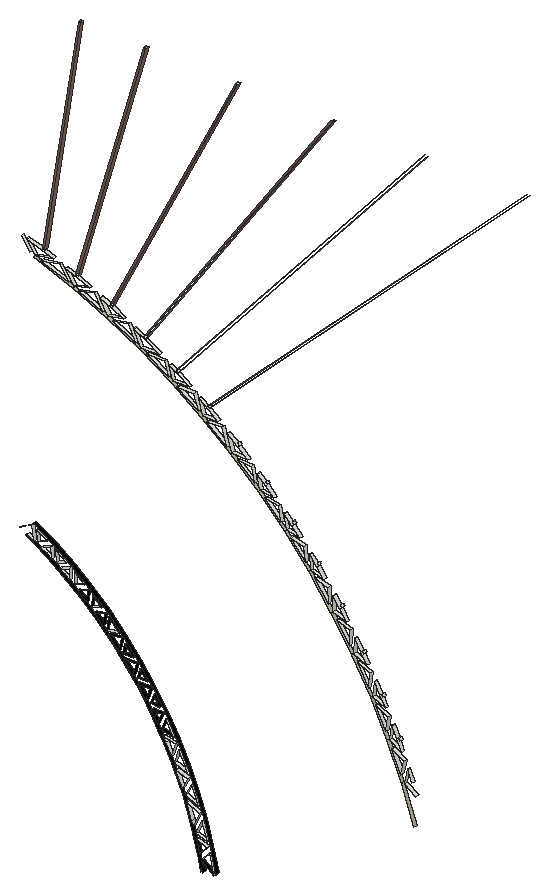
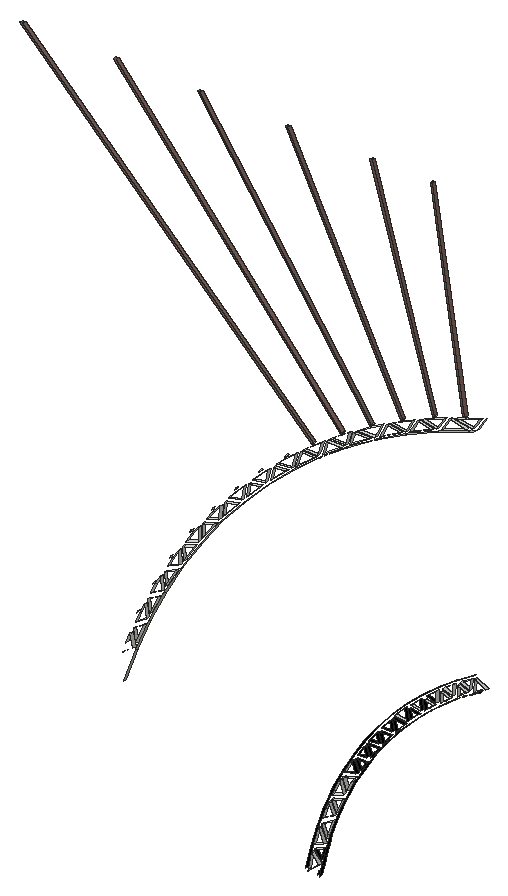
# SketchUp Ruby script. Lengths in inches.
U = 1.inch
M = Sketchup.active_model
def pt(a) = Geom::Point3d.new(a.map { |v| v * U })
def face(e, loops, mat)
  f = e.add_face(loops[0].map { |a| pt(a) })
  loops[1..].each { |l| e.add_face(l.map { |a| pt(a) }).erase! }
  f.material = f.back_material = mat if mat
  f
end
# faces: each face lists its corners as indices into pts; further lists are holes
def faces(e, pts, list, mat = nil) = list.each { |f| face(e, (f[0].is_a?(Array) ? f : [f]).map { |l| l.map { |i| pts[i] } }, mat) }
# xy, xz, yz: faces in a plane at the given z, y or x. An outline is a flat list of corners, or four numbers for a rectangle; further outlines are holes
def ring(l) = l.size == 4 ? [[l[0], l[1]], [l[2], l[1]], [l[2], l[3]], [l[0], l[3]]] : l.each_slice(2).to_a
def flat(e, list, mat, &to3) = list.each { |f| face(e, (f[0].is_a?(Array) ? f : [f]).map { |l| ring(l).map { |u, v| to3.(u, v) } }, mat) }
def xy(e, z, list, mat = nil) = flat(e, list, mat) { |x, y| [x, y, z] }
def xz(e, y, list, mat = nil) = flat(e, list, mat) { |x, z| [x, y, z] }
def yz(e, x, list, mat = nil) = flat(e, list, mat) { |y, z| [x, y, z] }
def lines(e, pts, list) = list.each { |a, b| e.add_line(pt(pts[a]), pt(pts[b])) }
# prism: a flat outline (further loops are holes) pulled along v
def prism(e, loops, v, mat = nil)
  f = face(e, loops, mat); d = Geom::Vector3d.new(v.map { |x| x * U })
  f.pushpull(f.normal.samedirection?(d) ? d.length : -d.length)
end
def box(e, o, s, mat = nil) = prism(e, [[o, [o[0] + s[0], o[1], o[2]], [o[0] + s[0], o[1] + s[1], o[2]], [o[0], o[1] + s[1], o[2]]]], [0, 0, s[2]], mat)
def at(x, y, z, deg = 0) = Geom::Transformation.translation(pt([x, y, z])) * Geom::Transformation.rotation(ORIGIN, Z_AXIS, deg.degrees)
def axes(o, x, y, z) = Geom::Transformation.new([*x, 0, *y, 0, *z, 0, *pt(o).to_a, 1])
def part(name) = M.definitions.add(name)
# library, detail: a bought-in or finely detailed component or shape, given as its bounding box
def library(name, o, s) = part(name).tap { |d| box(d.entities, o, s) }
def detail(e, o, s) = box(e.add_group.entities, o, s)
def put(e, d, t, mat = nil) = e.add_instance(d, t).tap { |i| i.material = mat if mat }
def group(e, t, mat = nil) = e.add_group.tap { |g| g.transformation = t; g.material = mat if mat }.entities
root = M.entities
M.materials.add("Tafisa-Terrarossa-PM780-4K").color = [148, 117, 107]
M.materials.add("Uniboard-L19-Putty-4K").color = [187, 181, 160]
M.materials.add("[Color M09]").color = [0, 0, 0]
xy(root,59.17,[[115.33,138,116.01,138.16]],"[Color M09]")
xy(root,59.41,[[115.33,138,115.86,138.16]],"[Color M09]")
xy(root,60.06,[[114.61,138,115.28,138.16]],"[Color M09]")
xy(root,60.3,[[114.58,138,115.15,138.16]],"[Color M09]")
xy(root,72.82,[[119,138,119.8,138.16]])
xy(root,73.01,[[118.79,138,119.59,138.16]])
xy(root,73.9,[[117.43,138,118.31,138.16]])
xy(root,74.1,[[117.19,138,118.07,138.16]])
xy(root,74.89,[[115.81,138,116.77,138.16]])
xy(root,75.08,[[115.51,138,116.49,138.16]])
xy(root,89.29,[[112.22,138,112.34,138.16],[115.67,138,115.8,138.16],[120.5,138,120.63,138.16],[125.54,138,125.68,138.16]])
yz(root,110.47,[[138,77.92,138.16,77.94]])
yz(root,112.11,[[138,77.33,138.16,77.35]])
yz(root,118.75,[[138,53.89,138.16,53.9]])
p = [[118.68,138,51.44],[118.55,138,52.01],[118.55,138.16,52.01],[118.68,138.16,51.44],[118.72,138,52.02],[119.36,138,51.48],
  [119.36,138.16,51.48],[118.72,138.16,52.02],[118.75,138,51.68],[118.8,138,51.47],[118.8,138.16,51.47],[118.75,138.16,51.68],
  [119.34,138,51.57],[119.34,138.16,51.57],[119.14,138,52.5],[119.14,138.16,52.5],[119.2,138,52.77],[119.47,138,51.6],
  [119.47,138.16,51.6],[119.2,138.16,52.77],[118.42,138,52.57],[118.42,138.16,52.57],[118.54,138,52.6],[118.62,138,52.28],
  [118.62,138.16,52.28],[118.54,138.16,52.6],[119,138,52.72],[119,138.16,52.72],[118.26,138,53.125],[118.26,138.16,53.125],
  [118.45,138,52.92],[118.45,138.16,52.92],[118.87,138,53.93],[118.87,138.16,53.93],[118.43,138,53.2],[119.02,138,52.97],
  [119.02,138.16,52.97],[118.43,138.16,53.2],[118.75,138,53.89],[118.75,138.16,53.89],[118.1,138,53.68],[118.1,138.16,53.68],
  [118.75,138,53.9],[118.75,138.16,53.9],[118.22,138,53.72],[118.29,138,53.48],[118.29,138.16,53.48],[118.22,138.16,53.72],
  [118.6,138,54.17],[118.6,138.16,54.17],[117.71,138,54.77],[117.71,138.16,54.77],[117.93,138,54.51],[117.93,138.16,54.51],
  [118.76,138,54.22],[118.76,138.16,54.22],[118.46,138,55.0625],[118.46,138.16,55.0625],[117.875,138,54.82],[118.54,138,54.48],
  [118.54,138.16,54.48],[117.875,138.16,54.82],[118.34,138,55.02],[118.34,138.16,55.02],[117.25,138,55.83],[117.25,138.16,55.83],
  [118.18,138,55.4],[118.18,138.16,55.4],[117.38,138,55.83],[117.72,138,55.05],[117.72,138.16,55.05],[117.38,138.16,55.83],
  [118.01,138,55.62],[118.01,138.16,55.62],[118.1875,138,55.6875],[118.1875,138.16,55.6875],[117.98,138,56.17],[117.98,138.16,56.17],
  [117.14,138,56.04],[117.14,138.16,56.04],[117.3,138,56.12],[117.96,138,55.89],[117.96,138.16,55.89],[117.3,138.16,56.12],
  [117.87,138,56.12],[117.87,138.16,56.12],[116.73,138,56.86],[116.73,138.16,56.86],[117.53,138,56.79],[117.53,138.16,56.79],
  [117.5,138,57.1],[117.5,138.16,57.1],[116.84,138,56.92],[117.12,138,56.36],[117.12,138.16,56.36],[116.84,138.16,56.92],
  [117.34,138,57.02],[117.34,138.16,57.02],[116.43,138,57.35],[116.43,138.16,57.35],[116.6875,138,57.17],[116.6875,138.16,57.17],
  [117.43,138,57.24],[117.43,138.16,57.24],[116.82,138,58.28],[116.82,138.16,58.28],[116.6,138,57.44],[117.26,138,57.29],
  [117.26,138.16,57.29],[116.6,138.16,57.44],[116.84,138,58.01],[116.84,138.16,58.01],[116.14,138,57.85],[116.14,138.16,57.85],
  [129.91,138,57.52],[129.25,138,59.34],[129.25,138.16,59.34],[129.91,138.16,57.52],[116.24,138,57.92],[116.41,138,57.63],
  [116.41,138.16,57.63],[116.24,138.16,57.92],[116.64,138,58.17],[116.64,138.16,58.17],[115.82,138,58.33],[115.82,138.16,58.33],
  [116.06,138,58.19],[116.06,138.16,58.19],[115.49,138,58.81],[115.49,138.16,58.81],[116.14,138,59.28],[116.14,138.16,59.28],
  [116.02,138,58.47],[116.53,138,58.44],[116.53,138.16,58.44],[116.02,138.16,58.47],[116.1875,138,58.95],[116.1875,138.16,58.95],
  [115.57,138,58.86],[115.79,138,58.53],[115.79,138.16,58.53],[115.57,138.16,58.86],[116.01,138,59.17],[116.01,138.16,59.17],
  [115.14,138,59.26],[115.14,138.16,59.26],[115.33,138,59.17],[115.33,138.16,59.17],[129.39,138,59.39],[130,138,58.98],
  [130,138.16,58.98],[129.39,138.16,59.39],[114.78,138,59.72],[114.78,138.16,59.72],[115.4,138,60.23],[115.4,138.16,60.23],
  [128.48,138,61.11],[128.48,138.16,61.11],[115.48,138,59.89],[115.33,138,59.41],[115.33,138.16,59.41],[115.48,138.16,59.89],
  [115.86,138,59.41],[115.86,138.16,59.41],[129.55,138,60.11],[129.55,138.16,60.11],[114.85,138,59.78],[115.1,138,59.46],
  [115.1,138.16,59.46],[114.85,138.16,59.78],[115.28,138,60.06],[115.28,138.16,60.06],[129.79,138,59.55],[129.79,138.16,59.55],
  [114.4,138,60.15],[114.4,138.16,60.15],[128.75,138,60.8125],[129.21,138,59.73],[129.21,138.16,59.73],[128.75,138.16,60.8125],
  [129.375,138,60.44],[129.375,138.16,60.44],[114.61,138,60.06],[114.61,138.16,60.06],[114.02,138,60.58],[114.02,138.16,60.58],
  [114.61,138,61.13],[114.61,138.16,61.13],[114.6875,138,60.82],[114.58,138,60.3],[114.58,138.16,60.3],[114.6875,138.16,60.82],
  [115.15,138,60.3],[115.15,138.16,60.3],[114.09,138,60.65],[114.35,138,60.35],[114.35,138.16,60.35],[114.09,138.16,60.65],
  [114.49,138,61.02],[114.49,138.16,61.02],[113.61,138,60.99],[113.61,138.16,60.99],[113.81,138,60.93],[113.81,138.16,60.93],
  [128.62,138,61.18],[129.25,138,60.8],[129.25,138.16,60.8],[128.62,138.16,61.18],[129.01,138,61.36],[129.01,138.16,61.36],
  [113.2,138,61.4],[113.2,138.16,61.4],[113.82,138,61.79],[113.72,138,61.1],[113.72,138.16,61.1],[113.82,138.16,61.79],
  [114.41,138,61.2],[114.41,138.16,61.2],[113.75,138,61.99],[113.75,138.16,61.99],[127.6,138,62.84],[127.6,138.16,62.84],
  [128.74,138,61.9],[128.74,138.16,61.9],[113.29,138,61.5],[113.52,138,61.27],[113.52,138.16,61.27],[113.29,138.16,61.5],
  [113.6,138,61.82],[113.6,138.16,61.82],[129.125,138,61.41],[129.17,138,61.3],[129.17,138.16,61.3],[129.125,138.16,61.41],
  [112.77,138,61.78],[112.77,138.16,61.78],[113.05,138,61.71],[113.05,138.16,61.71],[127.89,138,62.55],[128.42,138,61.51],
  [128.42,138.16,61.51],[127.89,138.16,62.55],[128.54,138,62.23],[128.54,138.16,62.23],[112.34,138,62.16],[112.34,138.16,62.16],
  [112.96,138,62.51],[112.91,138,61.95],[112.91,138.16,61.95],[112.96,138.16,62.51],[113.47,138,62.0625],[113.47,138.16,62.0625],
  [112.85,138,62.78],[112.85,138.16,62.78],[112.42,138,62.27],[112.66,138,62.06],[112.66,138.16,62.06],[112.42,138.16,62.27],
  [112.7,138,62.61],[112.7,138.16,62.61],[111.88,138,62.52],[111.88,138.16,62.52],[112.17,138,62.46],[112.17,138.16,62.46],
  [111.42,138,62.87],[111.42,138.16,62.87],[127.74,138,62.91],[128.39,138,62.58],[128.39,138.16,62.58],[127.74,138.16,62.91],
  [128.12,138,63.12],[128.12,138.16,63.12],[112.02,138,63.26],[112.01,138,62.69],[112.01,138.16,62.69],[112.02,138.16,63.26],
  [112.5625,138,62.84],[112.5625,138.16,62.84],[111.5,138,62.98],[111.75,138,62.78],[111.75,138.16,62.78],[111.5,138.16,62.98],
  [111.76,138,63.34],[111.76,138.16,63.34],[111.9,138,63.52],[111.9,138.16,63.52],[126.62,138,64.5],[126.62,138.16,64.5],
  [110.95,138,63.2],[110.95,138.16,63.2],[127.81,138,63.64],[127.81,138.16,63.64],[111.24,138,63.16],[111.24,138.16,63.16],
  [128.23,138,63.18],[128.28,138,63.07],[128.28,138.16,63.07],[128.23,138.16,63.18],[110.47,138,63.52],[110.47,138.16,63.52],
  [126.92,138,64.24],[127.52,138,63.23],[127.52,138.16,63.23],[126.92,138.16,64.24],[127.59,138,63.95],[127.59,138.16,63.95],
  [111.04,138,63.94],[111.07,138,63.38],[111.07,138.16,63.38],[111.04,138.16,63.94],[111.61,138,63.5625],[111.61,138.16,63.5625],
  [109.97,138,63.82],[109.97,138.16,63.82],[110.54,138,63.63],[110.8,138,63.45],[110.8,138.16,63.45],[110.54,138.16,63.63],
  [110.78,138,64.01],[110.78,138.16,64.01],[110.9,138,64.2],[110.9,138.16,64.2],[110.26,138,63.8],[110.26,138.16,63.8],
  [109.47,138,64.11],[109.47,138.16,64.11],[109.52,138,64.18],[109.87,138,63.97],[109.87,138.16,63.97],[109.52,138.16,64.18],
  [109.79,138,64.6875],[109.79,138.16,64.6875],[110.02,138,64.57],[110.08,138,64],[110.08,138.16,64],[110.02,138.16,64.57],
  [110.61,138,64.22],[110.61,138.16,64.22],[109.86,138,64.8125],[109.86,138.16,64.8125],[126.75,138,64.58],[127.42,138,64.29],
  [127.42,138.16,64.29],[126.75,138.16,64.58],[127.11,138,64.8125],[127.11,138.16,64.8125],[109.15,138,64.37],[109.15,138.16,64.37],
  [125.53,138,66.1],[125.53,138.16,66.1],[126.77,138,65.32],[126.77,138.16,65.32],[127.22,138,64.88],[127.28,138,64.78],
  [127.28,138.16,64.78],[127.22,138.16,64.88],[125.85,138,65.86],[126.51,138,64.88],[126.51,138.16,64.88],[125.85,138.16,65.86],
  [126.53,138,65.61],[126.53,138.16,65.61],[125.65,138,66.19],[126.35,138,65.94],[126.35,138.16,65.94],[125.65,138.16,66.19],
  [126.01,138,66.44],[126.01,138.16,66.44],[124.35,138,67.63],[124.35,138.16,67.63],[125.63,138,66.92],[125.63,138.16,66.92],
  [124.68,138,67.41],[125.4,138,66.48],[125.4,138.16,66.48],[124.68,138.16,67.41],[125.38,138,67.21],[125.38,138.16,67.21],
  [126.03,138,66.61],[126.11,138,66.52],[126.11,138.16,66.52],[126.03,138.16,66.61],[126.06,138,66.625],[126.06,138.16,66.625],
  [124.46,138,67.73],[125.17,138,67.52],[125.17,138.16,67.52],[124.46,138.16,67.73],[124.8,138,68],[124.8,138.16,68],
  [123.07,138,69.08],[123.07,138.16,69.08],[124.4,138,68.46],[124.4,138.16,68.46],[123.41,138,68.88],[124.1875,138,68],
  [124.1875,138.16,68],[123.41,138.16,68.88],[124.12,138,68.72],[124.12,138.16,68.72],[124.8125,138,68.17],[124.89,138,68.08],
  [124.89,138.16,68.08],[124.8125,138.16,68.17],[124.84,138,68.1875],[124.84,138.16,68.1875],[123.18,138,69.18],[123.89,138,69.03],
  [123.89,138.16,69.03],[123.18,138.16,69.18],[123.49,138,69.48],[123.49,138.16,69.48],[121.7,138,70.45],[121.7,138.16,70.45],
  [123.06,138,69.91],[123.06,138.16,69.91],[122.06,138,70.27],[122.89,138,69.4375],[122.89,138.16,69.4375],[122.06,138.16,70.27],
  [122.78,138,70.16],[122.78,138.16,70.16],[123.5,138,69.65],[123.58,138,69.57],[123.58,138.16,69.57],[123.5,138.16,69.65],
  [123.52,138,69.67],[123.52,138.16,69.67],[120.25,138,71.73],[120.25,138.16,71.73],[121.8,138,70.56],[122.53,138,70.45],
  [122.53,138.16,70.45],[121.8,138.16,70.56],[122.1,138,70.875],[122.1,138.16,70.875],[121.64,138,71.28],[121.64,138.16,71.28],
  [120.61,138,71.57],[121.5,138,70.79],[121.5,138.16,70.79],[120.61,138.16,71.57],[121.34,138,71.5],[121.34,138.16,71.5],
  [122.12,138,71.0625],[122.09,138,71.05],[122.09,138.16,71.05],[122.12,138.16,71.0625],[122.18,138,70.97],[122.18,138.16,70.97],
  [118.72,138,72.91],[118.72,138.16,72.91],[120.32,138,71.82],[121.16,138,71.74],[121.16,138.16,71.74],[120.32,138.16,71.82],
  [120.64,138,72.2],[120.64,138.16,72.2],[120.06,138,72.65],[120.06,138.16,72.65],[119,138,72.82],[120.0625,138,71.99],
  [120.0625,138.16,71.99],[119,138.16,72.82],[119.8,138,72.82],[119.8,138.16,72.82],[120.625,138,72.36],[120.6,138,72.35],
  [120.6,138.16,72.35],[120.625,138.16,72.36],[120.7,138,72.27],[120.7,138.16,72.27],[117.12,138,74],[117.12,138.16,74],
  [118.55,138,73.77],[118.79,138,73.01],[118.79,138.16,73.01],[118.55,138.16,73.77],[119.59,138,73.01],[119.08,138,73.41],
  [119.08,138.16,73.41],[119.59,138.16,73.01],[117.43,138,73.9],[118.54,138,73.15],[118.54,138.16,73.15],[117.43,138.16,73.9],
  [118.31,138,73.9],[118.31,138.16,73.9],[119.04,138,73.56],[119.14,138,73.49],[119.14,138.16,73.49],[119.04,138.16,73.56],
  [135.86,138,89.29],[135.86,138.16,89.29],[119.05,138,73.57],[119.05,138.16,73.57],[135.69,138,89.29],[135.69,138.16,89.29],
  [115.45,138,74.99],[115.45,138.16,74.99],[117,138,74.78],[117.19,138,74.1],[117.19,138.16,74.1],[117,138.16,74.78],
  [118.07,138,74.1],[117.45,138,74.52],[117.45,138.16,74.52],[118.07,138.16,74.1],[115.81,138,74.89],[116.96,138,74.21],
  [116.96,138.16,74.21],[115.81,138.16,74.89],[116.77,138,74.89],[116.77,138.16,74.89],[117.4,138,74.66],[117.5,138,74.6],
  [117.5,138.16,74.6],[117.4,138.16,74.66],[130.5,138,89.29],[130.5,138.16,89.29],[117.41,138,74.68],[117.41,138.16,74.68],
  [130.34,138,89.29],[130.34,138.16,89.29],[113.73,138,75.86],[113.73,138.16,75.86],[115.13,138,75.84],[115.51,138,75.08],
  [115.51,138.16,75.08],[115.13,138.16,75.84],[116.49,138,75.08],[115.75,138,75.52],[115.75,138.16,75.52],[116.49,138.16,75.08],
  [114.04,138,75.82],[115.23,138,75.21],[115.23,138.16,75.21],[114.04,138.16,75.82],[114.86,138,75.95],[114.86,138.16,75.95],
  [115.6875,138,75.66],[115.8,138,75.61],[115.8,138.16,75.61],[115.6875,138.16,75.66],[125.68,138,89.29],[125.68,138.16,89.29],
  [115.7,138,75.68],[115.7,138.16,75.68],[125.54,138,89.29],[125.54,138.16,89.29],[111.95,138,76.63],[111.95,138.16,76.63],
  [113.36,138,76.69],[113.78,138,75.97],[113.78,138.16,75.97],[113.36,138.16,76.69],[114.61,138,76.1],[114.61,138.16,76.1],
  [112.26,138,76.6],[113.5,138,76.07],[113.5,138.16,76.07],[112.26,138.16,76.6],[113.08,138,76.79],[113.08,138.16,76.79],
  [113.99,138,76.42],[113.99,138.16,76.42],[113.92,138,76.55],[114.03,138,76.51],[114.03,138.16,76.51],[113.92,138.16,76.55],
  [120.63,138,89.29],[120.63,138.16,89.29],[110.13,138,77.29],[110.13,138.16,77.29],[113.9375,138,76.58],[113.9375,138.16,76.58],
  [120.5,138,89.29],[120.5,138.16,89.29],[111.53,138,77.4375],[112,138,76.74],[112,138.16,76.74],[111.53,138.16,77.4375],
  [112.8125,138,76.93],[112.8125,138.16,76.93],[110.27,138,77.34],[111.71,138,76.82],[111.71,138.16,76.82],[110.27,138.16,77.34],
  [111.24,138,77.52],[111.24,138.16,77.52],[112.18,138,77.2],[112.18,138.16,77.2],[109.87,138,77.36],[109.87,138.16,77.36],
  [112.11,138,77.33],[112.22,138,77.29],[112.22,138.16,77.29],[112.11,138.16,77.33],[115.67,138,89.29],[112.11,138,77.35],
  [112.11,138.16,77.35],[115.67,138.16,89.29],[115.8,138,89.29],[115.8,138.16,89.29],[109.64,138,77.53],[109.23,138,78.16],
  [109.23,138.16,78.16],[109.64,138.16,77.53],[109.49,138,78.11],[109.92,138,77.47],[109.92,138.16,77.47],[109.49,138.16,78.11],
  [110.92,138,77.66],[110.92,138.16,77.66],[110.32,138,77.87],[110.32,138.16,77.87],[110.35,138,77.96],[110.47,138,77.92],
  [110.47,138.16,77.92],[110.35,138.16,77.96],[110.47,138,77.94],[112.33,138,89.27],[112.33,138.16,89.27],[110.47,138.16,77.94],
  [112.22,138,89.29],[112.22,138.16,89.29],[112.34,138,89.29],[112.34,138.16,89.29]]
faces(root,p,[[0,1,2,3],[4,5,6,7],[8,9,10,11],[16,17,18,19],[1,20,21,2],[22,23,24,25],[23,26,27,24],[20,28,29,21],
  [30,22,25,31],[32,16,19,33],[28,40,41,29],[40,50,51,41],[54,32,33,55],[56,54,55,57],[50,64,65,51],[74,56,57,75],
  [76,74,75,77],[64,78,79,65],[78,86,87,79],[90,76,77,91],[86,98,99,87],[102,90,91,103],[104,102,103,105],[106,107,108,109],
  [98,112,113,99],[110,106,109,111],[118,119,120,121],[119,122,123,120],[112,124,125,113],[126,118,121,127],[122,126,127,123],[124,128,129,125],
  [130,104,105,131],[132,133,134,135],[133,136,137,134],[138,139,140,141],[139,142,143,140],[136,132,135,137],[128,144,145,129],[146,138,141,147],
  [144,152,153,145],[154,130,131,155],[158,159,160,161],[162,158,161,163],[166,167,168,169],[167,170,171,168],[152,174,175,153],[182,166,169,183],
  [174,184,185,175],[186,154,155,187],[188,189,190,191],[192,188,191,193],[194,195,196,197],[195,198,199,196],[184,200,201,185],[202,194,197,203],
  [198,202,203,199],[200,210,211,201],[212,213,214,215],[218,186,187,219],[216,212,215,217],[224,225,226,227],[225,228,229,226],[210,234,235,211],
  [236,224,227,237],[228,236,237,229],[234,244,245,235],[246,247,248,249],[252,218,219,253],[254,255,256,257],[255,258,259,256],[250,246,249,251],
  [244,260,261,245],[262,254,257,263],[260,264,265,261],[273,276,277,274],[284,252,253,285],[264,288,289,265],[288,298,299,289],[298,312,313,299],
  [320,284,285,321],[312,324,325,313],[338,320,321,339]],"[Color M09]")
faces(root,p,[[5,12,13,6],[12,14,15,13],[14,4,7,15],[26,30,31,27],[34,35,36,37],[35,38,39,36],[42,34,37,43],[44,45,46,47],
  [45,48,49,46],[52,44,47,53],[48,52,53,49],[58,59,60,61],[59,62,63,60],[66,58,61,67],[62,66,67,63],[68,69,70,71],
  [69,72,73,70],[72,68,71,73],[80,81,82,83],[81,84,85,82],[88,80,83,89],[84,88,89,85],[92,93,94,95],[93,96,97,94],
  [100,92,95,101],[96,100,101,97],[107,110,111,108],[148,149,150,151],[164,148,151,165],[172,164,165,173],[176,177,178,179],[177,180,181,178],
  [180,176,179,181],[204,205,206,207],[205,208,209,206],[213,216,217,214],[222,204,207,223],[230,231,232,233],[208,222,223,209],[238,239,240,241],
  [239,242,243,240],[247,250,251,248],[242,238,241,243],[258,262,263,259],[266,267,268,269],[267,270,271,268],[272,273,274,275],[278,279,280,281],
  [279,282,283,280],[276,272,275,277],[290,266,269,291],[292,278,281,293],[270,290,291,271],[294,295,296,297],[282,292,293,283],[300,301,302,303],
  [301,304,305,302],[306,307,308,309],[307,310,311,308],[314,315,316,317],[315,318,319,316],[322,314,317,323],[310,306,309,311],[318,322,323,319],
  [326,327,328,329],[327,330,331,328],[332,333,334,335],[333,336,337,334],[304,300,303,305],[336,332,335,337],[340,341,342,343],[341,344,345,342],
  [330,346,347,331],[350,340,343,351],[344,350,351,345],[352,353,354,355],[356,357,358,359],[357,360,361,358],[360,356,359,361],[362,363,364,365],
  [363,366,367,364],[370,362,365,371],[366,370,371,367],[372,373,374,375],[373,376,377,374],[378,379,380,381],[382,378,381,383],[376,372,375,377],
  [384,385,386,387],[385,388,389,386],[392,384,387,393],[394,395,396,397],[395,398,399,396],[388,392,393,389],[400,401,402,403],[404,400,403,405],
  [398,394,397,399],[406,407,408,409],[407,410,411,408],[414,406,409,415],[416,417,418,419],[417,420,421,418],[410,414,415,411],[422,423,424,425],
  [426,422,425,427],[420,416,419,421],[430,431,432,433],[431,434,435,432],[436,430,433,437],[438,439,440,441],[439,442,443,440],[434,436,437,435],
  [444,445,446,447],[445,448,449,446],[442,438,441,443],[452,453,454,455],[453,456,457,454],[458,452,455,459],[460,461,462,463],[461,464,465,462],
  [456,458,459,457],[466,467,468,469],[467,470,471,468],[474,475,476,477],[478,479,480,481],[482,483,484,485],[483,486,487,484],[479,474,477,480],
  [488,489,490,491],[494,488,491,495],[500,501,502,503],[504,505,506,507],[508,509,510,511],[509,512,513,510],[505,500,503,506],[514,515,516,517],
  [520,514,517,521],[526,527,528,529],[530,531,532,533],[534,535,536,537],[535,538,539,536],[531,526,529,532],[540,541,542,543],[546,540,543,547],
  [538,534,537,539],[552,553,554,555],[553,556,557,554],[558,559,560,561],[559,562,563,560],[556,564,565,557],[564,552,555,565],[566,567,568,569],
  [562,558,561,563],[574,566,569,575],[578,579,580,581],[579,582,583,580],[584,585,586,587],[585,588,589,586],[582,590,591,583],[590,578,581,591],
  [588,584,587,589],[594,595,596,597],[604,605,606,607],[608,609,610,611],[609,612,613,610],[612,614,615,613],[614,608,611,615],[616,617,618,619],
  [621,626,627,622]])
faces(root,p,[[114,115,116,117],[115,156,157,116],[156,220,221,157],[220,286,287,221],[286,348,349,287],[348,368,369,349],[368,390,391,369],[390,412,413,391],
  [412,428,429,413],[428,450,451,429],[450,472,473,451],[472,498,499,473],[498,524,525,499],[524,550,551,525],[550,572,573,551],[572,592,593,573]],"Uniboard-L19-Putty-4K")
faces(root,p,[[489,492,493,490],[496,494,495,497],[515,518,519,516],[522,520,521,523],[541,544,545,542],[548,546,547,549],[567,570,571,568],[576,574,575,577],
  [598,599,600,601],[595,602,603,596],[620,621,622,623],[624,616,619,625]],"Tafisa-Terrarossa-PM780-4K")
